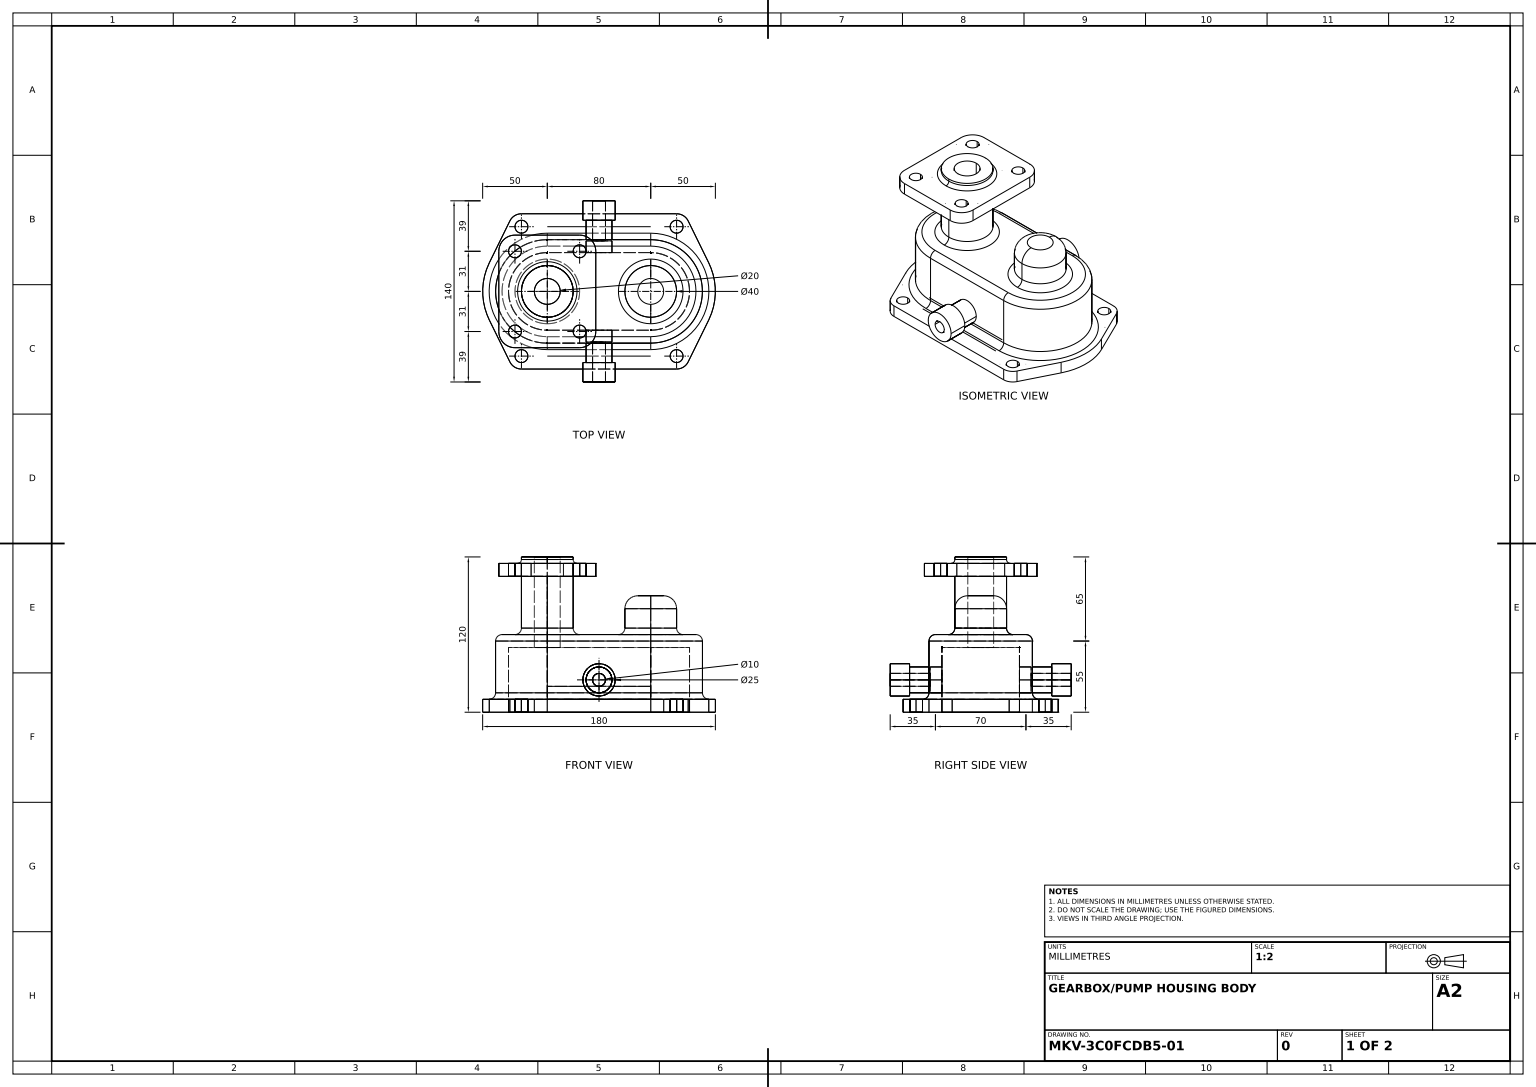
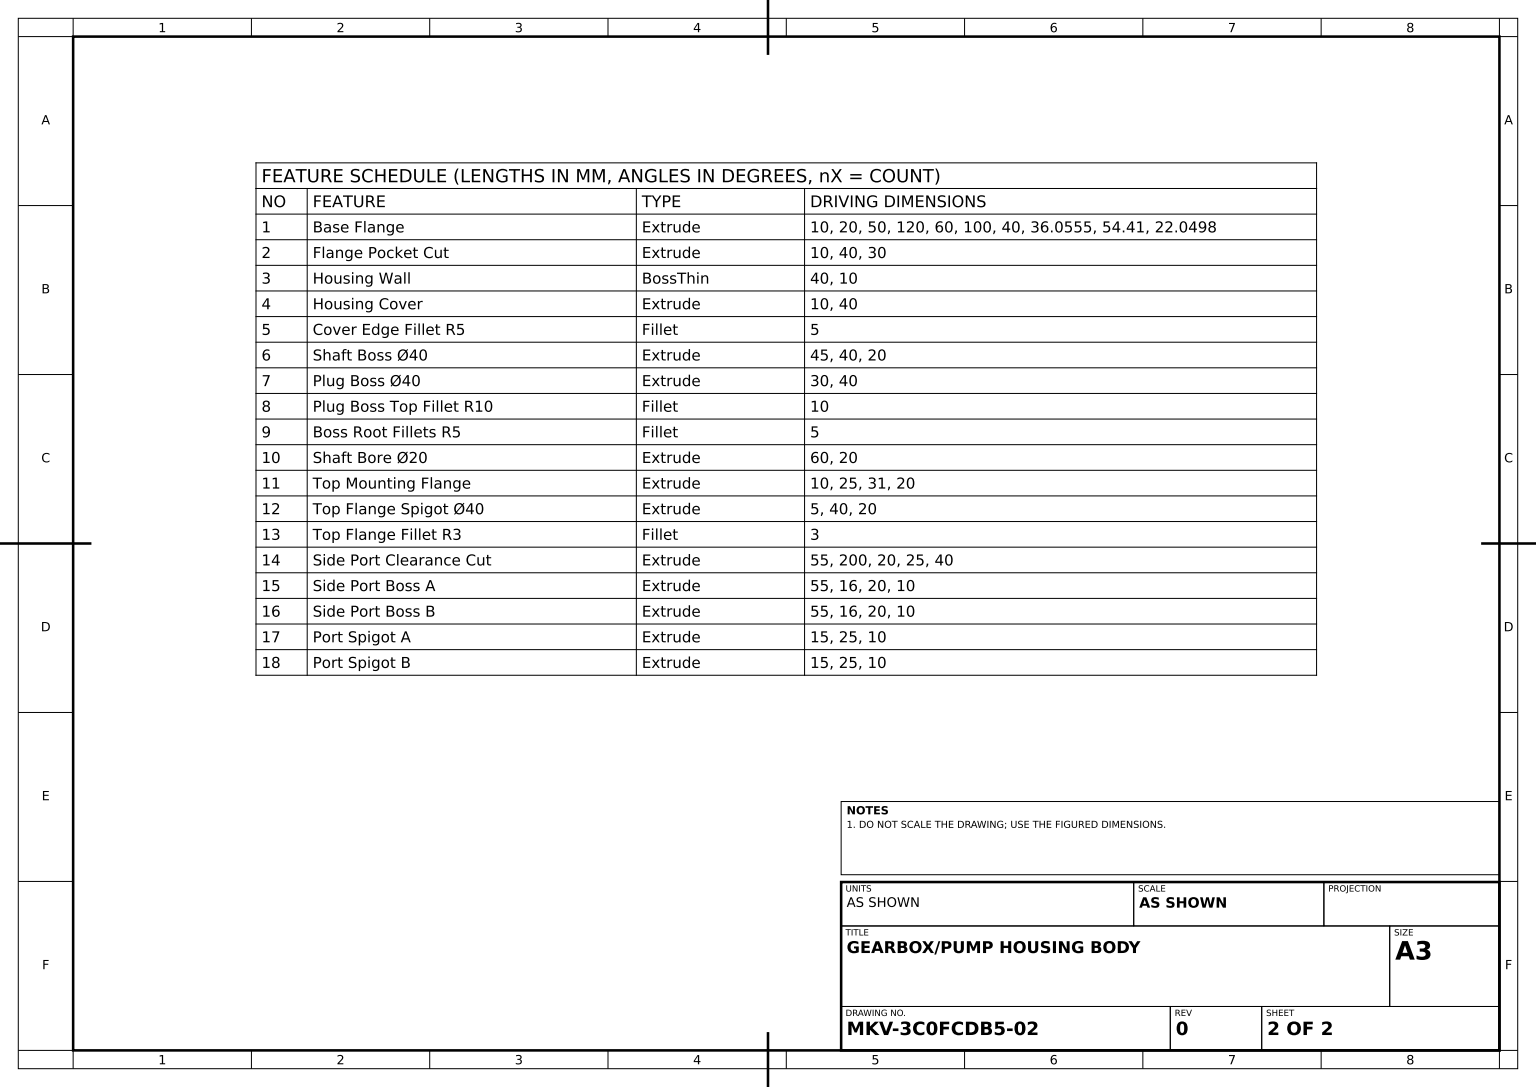
solid
v1 (-5,25,70)
v2 (5,25,70)
e1 v1 v2 CIRCLE(AX(P(0,25,70),D(0,0,1),D(1,0,0)),5)
v3 (5,25,39)
e2 v3 v2 LINE
v4 (-5,25,39)
e3 v4 v3 CIRCLE(AX(P(0,25,39),D(0,0,1),D(1,0,0)),5)
e4 v4 v1 LINE
face CYL(AX(P(0,25,39),D(0,0,1),D(1,0,0)),5) rev [e1 -e2 -e3 e4]
v5 (40,60,-35)
v6 (-40,60,-35)
e5 v5 v6 LINE
v7 (40,55,-40)
e6 v5 v7 CIRCLE(AX(P(40,55,-35),D(-1,0,0),D(0,0,1)),5)
v8 (-40,55,-40)
e7 v8 v7 LINE
e8 v6 v8 CIRCLE(AX(P(-40,55,-35),D(-1,0,0),D(0,0,1)),5)
face CYL(AX(P(-40,55,-35),D(1,0,0),D(0,0,-1)),5) [-e5 e6 -e7 -e8]
v9 (-60,10,55)
v10 (-60,0,55)
e9 v9 v10 LINE
v11 (-60,0,45)
e10 v11 v10 CIRCLE(AX(P(-60,0,50),D(0,1,0),D(0,0,1)),5)
v12 (-60,10,45)
e11 v12 v11 LINE
e12 v12 v9 CIRCLE(AX(P(-60,10,50),D(0,1,0),D(0,0,1)),5)
face CYL(AX(P(-60,10,50),D(0,-1,0),D(0,0,-1)),5) rev [e9 -e10 -e11 e12]
v13 (40,15,-40)
e13 v7 v13 LINE
v14 (40,55,40)
e14 v7 v14 CIRCLE(AX(P(40,55,0),D(0,-1,0),D(0,0,1)),40)
v15 (40,15,40)
e15 v14 v15 LINE
e16 v15 v13 CIRCLE(AX(P(40,15,0),D(0,1,0),D(0,0,1)),40)
face CYL(AX(P(40,50,0),D(0,-1,0),D(0,0,-1)),40) [-e13 e14 e15 e16]
v16 (-68.975088,0,-54.409965)
v17 (-84.875442,0,-22.049823)
e17 v16 v17 LINE
v18 (-84.875442,10,-22.049823)
e18 v18 v17 LINE
v19 (-68.975088,10,-54.409965)
e19 v19 v18 LINE
e20 v19 v16 LINE
face PLANE(AX(P(-84.875442,10,-22.049823),D(0.897508841,0,0.440996464),D(0.440996464,0,-0.897508841))) rev [e17 -e18 -e19 e20]
v20 (-40,115,23)
v21 (-40,115,-23)
e21 v20 v21 CIRCLE(AX(P(-40,115,0),D(0,-1,0),D(0,0,1)),23)
v22 (-40,118,20)
e22 v22 v20 CIRCLE(AX(P(-40,118,23),D(-1,0,0),D(0,0,1)),3)
v23 (-40,118,-20)
e23 v23 v22 CIRCLE(AX(P(-40,118,0),D(0,1,0),D(0,0,1)),20)
e24 v23 v21 CIRCLE(AX(P(-40,118,-23),D(1,0,0),D(0,0,-1)),3)
face TORUS(AX(P(-40,118,0),D(0,1,0),D(0,0,1)),23,3) rev [-e21 -e22 -e23 e24]
v24 (10,25,30)
v25 (-10,25,30)
e25 v24 v25 CIRCLE(AX(P(0,25,30),D(0,0,1),D(1,0,0)),10)
v26 (10,25,39)
e26 v24 v26 LINE
v27 (-10,25,39)
e27 v27 v26 CIRCLE(AX(P(0,25,39),D(0,0,-1),D(1,0,0)),10)
e28 v25 v27 LINE
face CYL(AX(P(0,25,-145),D(0,0,1),D(1,0,0)),10) rev [-e25 e26 -e27 -e28]
v28 (40,10,-45)
v29 (40,10,45)
e29 v28 v29 CIRCLE(AX(P(40,10,0),D(0,-1,0),D(0,0,1)),45)
v30 (-40,10,45)
e30 v29 v30 LINE
v31 (-40,10,-45)
e31 v30 v31 CIRCLE(AX(P(-40,10,0),D(0,-1,0),D(0,0,1)),45)
e32 v31 v28 LINE
v32 (60,10,-45)
v33 (60,10,-55)
e33 v32 v33 CIRCLE(AX(P(60,10,-50),D(0,1,0),D(0,0,1)),5)
e34 v33 v32 CIRCLE(AX(P(60,10,-50),D(0,1,0),D(0,0,1)),5)
e35 v9 v12 CIRCLE(AX(P(-60,10,50),D(0,1,0),D(0,0,1)),5)
v34 (60,10,45)
v35 (60,10,55)
e36 v34 v35 CIRCLE(AX(P(60,10,50),D(0,1,0),D(0,0,1)),5)
e37 v35 v34 CIRCLE(AX(P(60,10,50),D(0,1,0),D(0,0,1)),5)
v36 (60,10,60)
v37 (68.975088,10,54.409965)
e38 v36 v37 CIRCLE(AX(P(60,10,50),D(0,1,0),D(0,0,1)),10)
v38 (84.875442,10,22.049823)
e39 v37 v38 LINE
v39 (84.875442,10,-22.049823)
e40 v38 v39 CIRCLE(AX(P(40,10,0),D(0,1,0),D(0,0,1)),50)
v40 (68.975088,10,-54.409965)
e41 v39 v40 LINE
v41 (60,10,-60)
e42 v40 v41 CIRCLE(AX(P(60,10,-50),D(0,1,0),D(0,0,1)),10)
v42 (-60,10,-60)
e43 v41 v42 LINE
e44 v42 v19 CIRCLE(AX(P(-60,10,-50),D(0,1,0),D(0,0,1)),10)
v43 (-84.875442,10,22.049823)
e45 v18 v43 CIRCLE(AX(P(-40,10,0),D(0,1,0),D(0,0,1)),50)
v44 (-68.975088,10,54.409965)
e46 v43 v44 LINE
v45 (-60,10,60)
e47 v44 v45 CIRCLE(AX(P(-60,10,50),D(0,1,0),D(0,0,1)),10)
e48 v45 v36 LINE
v46 (-60,10,-55)
v47 (-60,10,-45)
e49 v46 v47 CIRCLE(AX(P(-60,10,-50),D(0,1,0),D(0,0,1)),5)
e50 v47 v46 CIRCLE(AX(P(-60,10,-50),D(0,1,0),D(0,0,1)),5)
face PLANE(AX(P(-60,10,-50),D(0,1,0),D(0,0,1))) [e29 e30 e31 e32] [-e33 -e34] [-e35 -e12] [-e36 -e37] [e38 e39 e40 e41 e42 e43 e44 e19 e45 e46 e47 e48] [-e49 -e50]
v48 (-15,105,-26)
v49 (-15,105,-36)
e51 v48 v49 CIRCLE(AX(P(-15,105,-31),D(0,1,0),D(0,0,1)),5)
e52 v49 v48 CIRCLE(AX(P(-15,105,-31),D(0,1,0),D(0,0,1)),5)
v50 (-40,105,20)
v51 (-40,105,-20)
e53 v50 v51 CIRCLE(AX(P(-40,105,0),D(0,1,0),D(0,0,1)),20)
e54 v51 v50 CIRCLE(AX(P(-40,105,0),D(0,1,0),D(0,0,1)),20)
v52 (-65,105,26)
v53 (-65,105,36)
e55 v52 v53 CIRCLE(AX(P(-65,105,31),D(0,1,0),D(0,0,1)),5)
e56 v53 v52 CIRCLE(AX(P(-65,105,31),D(0,1,0),D(0,0,1)),5)
v54 (-77.5,105,31)
v55 (-65,105,43.5)
e57 v54 v55 CIRCLE(AX(P(-65,105,31),D(0,1,0),D(0,0,1)),12.5)
v56 (-77.5,105,-31)
e58 v56 v54 LINE
v57 (-65,105,-43.5)
e59 v57 v56 CIRCLE(AX(P(-65,105,-31),D(0,1,0),D(0,0,1)),12.5)
v58 (-15,105,-43.5)
e60 v58 v57 LINE
v59 (-2.5,105,-31)
e61 v59 v58 CIRCLE(AX(P(-15,105,-31),D(0,1,0),D(0,0,1)),12.5)
v60 (-2.5,105,31)
e62 v60 v59 LINE
v61 (-15,105,43.5)
e63 v61 v60 CIRCLE(AX(P(-15,105,31),D(0,1,0),D(0,0,1)),12.5)
e64 v55 v61 LINE
v62 (-65,105,-26)
v63 (-65,105,-36)
e65 v62 v63 CIRCLE(AX(P(-65,105,-31),D(0,1,0),D(0,0,1)),5)
e66 v63 v62 CIRCLE(AX(P(-65,105,-31),D(0,1,0),D(0,0,1)),5)
v64 (-15,105,36)
v65 (-15,105,26)
e67 v64 v65 CIRCLE(AX(P(-15,105,31),D(0,1,0),D(0,0,1)),5)
e68 v65 v64 CIRCLE(AX(P(-15,105,31),D(0,1,0),D(0,0,1)),5)
face PLANE(AX(P(-65,105,-31),D(0,1,0),D(0,0,1))) rev [e51 e52] [e53 e54] [e55 e56] [-e57 -e58 -e59 -e60 -e61 -e62 -e63 -e64] [e65 e66] [e67 e68]
v66 (60,0,60)
v67 (68.975088,0,54.409965)
e69 v66 v67 CIRCLE(AX(P(60,0,50),D(0,1,0),D(0,0,1)),10)
e70 v37 v67 LINE
e71 v36 v66 LINE
face CYL(AX(P(60,10,50),D(0,-1,0),D(0,0,-1)),10) [e69 -e70 -e38 e71]
v68 (-60,0,60)
e72 v45 v68 LINE
e73 v68 v66 LINE
face PLANE(AX(P(-60,10,60),D(0,0,-1),D(-1,0,0))) rev [-e48 e72 e73 -e71]
v69 (68.975088,0,-54.409965)
e74 v40 v69 LINE
v70 (84.875442,0,-22.049823)
e75 v39 v70 LINE
e76 v70 v69 LINE
face PLANE(AX(P(84.875442,10,-22.049823),D(-0.897508841,0,0.440996464),D(0.440996464,0,0.897508841))) rev [-e74 -e41 e75 e76]
v71 (-60,0,-45)
v72 (-60,0,-55)
e77 v71 v72 CIRCLE(AX(P(-60,0,-50),D(0,1,0),D(0,0,1)),5)
e78 v47 v71 LINE
e79 v46 v72 LINE
face CYL(AX(P(-60,10,-50),D(0,-1,0),D(0,0,-1)),5) rev [-e77 -e78 e50 e79]
v73 (-40,50,10)
v74 (-40,50,-10)
e80 v73 v74 CIRCLE(AX(P(-40,50,0),D(0,1,0),D(0,0,1)),10)
v75 (-40,120,10)
e81 v75 v73 LINE
v76 (-40,120,-10)
e82 v75 v76 CIRCLE(AX(P(-40,120,0),D(0,1,0),D(0,0,1)),10)
e83 v76 v74 LINE
face CYL(AX(P(-40,105,0),D(0,-1,0),D(0,0,-1)),10) rev [-e80 -e81 e82 e83]
e84 v25 v24 CIRCLE(AX(P(0,25,30),D(0,0,1),D(1,0,0)),10)
e85 v26 v27 CIRCLE(AX(P(0,25,39),D(0,0,-1),D(1,0,0)),10)
face CYL(AX(P(0,25,-145),D(0,0,1),D(1,0,0)),10) rev [-e26 -e84 e28 -e85]
v77 (60,0,-60)
e86 v41 v77 LINE
e87 v69 v77 CIRCLE(AX(P(60,0,-50),D(0,1,0),D(0,0,1)),10)
face CYL(AX(P(60,10,-50),D(0,-1,0),D(0,0,-1)),10) [-e86 -e42 e74 e87]
v78 (-40,15,-40)
e88 v78 v31 CIRCLE(AX(P(-40,15,-45),D(1,0,0),D(0,0,-1)),5)
v79 (-40,15,40)
e89 v30 v79 CIRCLE(AX(P(-40,15,45),D(1,0,0),D(0,0,-1)),5)
e90 v78 v79 CIRCLE(AX(P(-40,15,0),D(0,1,0),D(0,0,1)),40)
face TORUS(AX(P(-40,15,0),D(0,1,0),D(0,0,1)),45,5) rev [e88 -e31 e89 -e90]
v80 (-40,120,20)
v81 (-40,120,-20)
e91 v80 v81 CIRCLE(AX(P(-40,120,0),D(0,1,0),D(0,0,1)),20)
e92 v80 v22 LINE
e93 v22 v23 CIRCLE(AX(P(-40,118,0),D(0,1,0),D(0,0,1)),20)
e94 v81 v23 LINE
face CYL(AX(P(-40,120,0),D(0,-1,0),D(0,0,-1)),20) [-e91 e92 e93 -e94]
v82 (40,60,35)
e95 v82 v5 CIRCLE(AX(P(40,60,0),D(0,1,0),D(0,0,1)),35)
e96 v14 v82 CIRCLE(AX(P(40,55,35),D(-1,0,0),D(0,0,1)),5)
face TORUS(AX(P(40,55,0),D(0,1,0),D(0,0,1)),35,5) [-e6 -e95 -e96 -e14]
v83 (40,80,-20)
v84 (40,80,20)
e97 v83 v84 CIRCLE(AX(P(40,80,0),D(0,-1,0),D(0,0,1)),20)
v85 (40,90,-10)
e98 v83 v85 CIRCLE(AX(P(40,80,-10),D(1,0,0),D(0,0,-1)),10)
v86 (40,90,10)
e99 v86 v85 CIRCLE(AX(P(40,90,0),D(0,1,0),D(0,0,1)),10)
e100 v84 v86 CIRCLE(AX(P(40,80,10),D(-1,0,0),D(0,0,1)),10)
face TORUS(AX(P(40,80,0),D(0,1,0),D(0,0,1)),10,10) [-e97 e98 -e99 -e100]
v87 (-65,115,-43.5)
v88 (-77.5,115,-31)
e101 v87 v88 CIRCLE(AX(P(-65,115,-31),D(0,1,0),D(0,0,1)),12.5)
v89 (-77.5,115,31)
e102 v88 v89 LINE
v90 (-65,115,43.5)
e103 v89 v90 CIRCLE(AX(P(-65,115,31),D(0,1,0),D(0,0,1)),12.5)
v91 (-15,115,43.5)
e104 v90 v91 LINE
v92 (-2.5,115,31)
e105 v91 v92 CIRCLE(AX(P(-15,115,31),D(0,1,0),D(0,0,1)),12.5)
v93 (-2.5,115,-31)
e106 v92 v93 LINE
v94 (-15,115,-43.5)
e107 v93 v94 CIRCLE(AX(P(-15,115,-31),D(0,1,0),D(0,0,1)),12.5)
e108 v94 v87 LINE
e109 v21 v20 CIRCLE(AX(P(-40,115,0),D(0,-1,0),D(0,0,1)),23)
v95 (-65,115,26)
v96 (-65,115,36)
e110 v95 v96 CIRCLE(AX(P(-65,115,31),D(0,1,0),D(0,0,1)),5)
e111 v96 v95 CIRCLE(AX(P(-65,115,31),D(0,1,0),D(0,0,1)),5)
v97 (-15,115,36)
v98 (-15,115,26)
e112 v97 v98 CIRCLE(AX(P(-15,115,31),D(0,1,0),D(0,0,1)),5)
e113 v98 v97 CIRCLE(AX(P(-15,115,31),D(0,1,0),D(0,0,1)),5)
v99 (-65,115,-36)
v100 (-65,115,-26)
e114 v99 v100 CIRCLE(AX(P(-65,115,-31),D(0,1,0),D(0,0,1)),5)
e115 v100 v99 CIRCLE(AX(P(-65,115,-31),D(0,1,0),D(0,0,1)),5)
v101 (-15,115,-36)
v102 (-15,115,-26)
e116 v101 v102 CIRCLE(AX(P(-15,115,-31),D(0,1,0),D(0,0,1)),5)
e117 v102 v101 CIRCLE(AX(P(-15,115,-31),D(0,1,0),D(0,0,1)),5)
face PLANE(AX(P(-65,115,-31),D(0,1,0),D(0,0,1))) [e101 e102 e103 e104 e105 e106 e107 e108] [e109 e21] [-e110 -e111] [-e112 -e113] [-e114 -e115] [-e116 -e117]
v103 (60,0,45)
e118 v34 v103 LINE
v104 (60,0,55)
e119 v104 v103 CIRCLE(AX(P(60,0,50),D(0,1,0),D(0,0,1)),5)
e120 v35 v104 LINE
face CYL(AX(P(60,10,50),D(0,-1,0),D(0,0,-1)),5) rev [e118 -e119 -e120 e37]
e121 v92 v60 LINE
e122 v93 v59 LINE
face PLANE(AX(P(-2.5,115,-31),D(-1,0,0),D(0,0,1))) rev [-e106 e121 e62 -e122]
v105 (-40,65,-20)
v106 (-40,65,20)
e123 v105 v106 CIRCLE(AX(P(-40,65,0),D(0,1,0),D(0,0,1)),20)
v107 (-40,60,-25)
e124 v105 v107 CIRCLE(AX(P(-40,65,-25),D(1,0,0),D(0,0,-1)),5)
v108 (-40,60,25)
e125 v108 v107 CIRCLE(AX(P(-40,60,0),D(0,-1,0),D(0,0,1)),25)
e126 v106 v108 CIRCLE(AX(P(-40,65,25),D(-1,0,0),D(0,0,1)),5)
face TORUS(AX(P(-40,65,0),D(0,1,0),D(0,0,1)),25,5) rev [-e123 e124 -e125 -e126]
v109 (-5,25,-39)
v110 (5,25,-39)
e127 v109 v110 CIRCLE(AX(P(0,25,-39),D(0,0,1),D(1,0,0)),5)
e128 v110 v109 CIRCLE(AX(P(0,25,-39),D(0,0,1),D(1,0,0)),5)
v111 (-10,25,-39)
v112 (10,25,-39)
e129 v111 v112 CIRCLE(AX(P(0,25,-39),D(0,0,1),D(1,0,0)),10)
e130 v112 v111 CIRCLE(AX(P(0,25,-39),D(0,0,1),D(1,0,0)),10)
face PLANE(AX(P(0,25,-39),D(0,0,1),D(1,0,0))) [-e127 -e128] [e129 e130]
v113 (-84.875442,0,22.049823)
e131 v43 v113 LINE
e132 v17 v113 CIRCLE(AX(P(-40,0,0),D(0,1,0),D(0,0,1)),50)
face CYL(AX(P(-40,10,0),D(0,-1,0),D(0,0,-1)),50) [-e131 -e45 e18 e132]
v114 (-60,0,-60)
e133 v42 v114 LINE
e134 v114 v16 CIRCLE(AX(P(-60,0,-50),D(0,1,0),D(0,0,1)),10)
face CYL(AX(P(-60,10,-50),D(0,-1,0),D(0,0,-1)),10) [e133 e134 -e20 -e44]
v115 (-40,50,30)
v116 (40,50,30)
e135 v115 v116 LINE
v117 (-40,50,-30)
e136 v117 v115 CIRCLE(AX(P(-40,50,0),D(0,1,0),D(1,0,0)),30)
v118 (40,50,-30)
e137 v118 v117 LINE
e138 v116 v118 CIRCLE(AX(P(40,50,0),D(0,1,0),D(1,0,0)),30)
e139 v74 v73 CIRCLE(AX(P(-40,50,0),D(0,1,0),D(0,0,1)),10)
face PLANE(AX(P(-40,50,0),D(0,1,0),D(0,0,1))) rev [-e135 -e136 -e137 -e138] [e139 e80]
v119 (-5,25,-70)
e140 v109 v119 LINE
v120 (5,25,-70)
e141 v119 v120 CIRCLE(AX(P(0,25,-70),D(0,0,-1),D(-1,0,0)),5)
e142 v110 v120 LINE
face CYL(AX(P(0,25,-39),D(0,0,-1),D(-1,0,0)),5) rev [e128 e140 e141 -e142]
e143 v95 v52 LINE
e144 v96 v53 LINE
face CYL(AX(P(-65,115,31),D(0,-1,0),D(0,0,-1)),5) rev [-e55 -e143 e110 e144]
e145 v76 v75 CIRCLE(AX(P(-40,120,0),D(0,1,0),D(0,0,1)),10)
face CYL(AX(P(-40,105,0),D(0,-1,0),D(0,0,-1)),10) rev [e145 e81 -e139 -e83]
v121 (40,0,30)
e146 v121 v116 LINE
v122 (-40,0,30)
e147 v122 v121 LINE
e148 v122 v115 LINE
face PLANE(AX(P(-40,0,30),D(0,0,1),D(1,0,0))) rev [e84 e25] [-e146 -e147 e148 e135]
e149 v84 v83 CIRCLE(AX(P(40,80,0),D(0,-1,0),D(0,0,1)),20)
v123 (40,65,-20)
e150 v83 v123 LINE
v124 (40,65,20)
e151 v123 v124 CIRCLE(AX(P(40,65,0),D(0,1,0),D(0,0,1)),20)
e152 v84 v124 LINE
face CYL(AX(P(40,90,0),D(0,-1,0),D(0,0,-1)),20) [e149 e150 e151 -e152]
v125 (-40,55,40)
e153 v125 v8 CIRCLE(AX(P(-40,55,0),D(0,-1,0),D(0,0,1)),40)
v126 (-40,60,35)
e154 v125 v126 CIRCLE(AX(P(-40,55,35),D(-1,0,0),D(0,0,1)),5)
e155 v6 v126 CIRCLE(AX(P(-40,60,0),D(0,1,0),D(0,0,1)),35)
face TORUS(AX(P(-40,55,0),D(0,1,0),D(0,0,1)),35,5) [-e153 e154 -e155 e8]
v127 (-10,25,-30)
e156 v111 v127 LINE
v128 (10,25,-30)
e157 v112 v128 LINE
e158 v127 v128 CIRCLE(AX(P(0,25,-30),D(0,0,-1),D(-1,0,0)),10)
face CYL(AX(P(0,25,-145),D(0,0,1),D(1,0,0)),10) rev [-e156 -e130 e157 -e158]
v129 (40,60,-25)
e159 v123 v129 CIRCLE(AX(P(40,65,-25),D(1,0,0),D(0,0,-1)),5)
e160 v124 v123 CIRCLE(AX(P(40,65,0),D(0,1,0),D(0,0,1)),20)
v130 (40,60,25)
e161 v124 v130 CIRCLE(AX(P(40,65,25),D(-1,0,0),D(0,0,1)),5)
e162 v129 v130 CIRCLE(AX(P(40,60,0),D(0,-1,0),D(0,0,1)),25)
face TORUS(AX(P(40,65,0),D(0,1,0),D(0,0,1)),25,5) rev [-e159 -e160 e161 -e162]
e163 v107 v108 CIRCLE(AX(P(-40,60,0),D(0,-1,0),D(0,0,1)),25)
e164 v106 v105 CIRCLE(AX(P(-40,65,0),D(0,1,0),D(0,0,1)),20)
face TORUS(AX(P(-40,65,0),D(0,1,0),D(0,0,1)),25,5) rev [e126 -e163 -e124 -e164]
e165 v125 v79 LINE
e166 v8 v78 LINE
face CYL(AX(P(-40,50,0),D(0,-1,0),D(0,0,-1)),40) [e90 -e165 e153 e166]
e167 v130 v129 CIRCLE(AX(P(40,60,0),D(0,-1,0),D(0,0,1)),25)
face TORUS(AX(P(40,65,0),D(0,1,0),D(0,0,1)),25,5) rev [-e167 -e161 -e151 e159]
v131 (60,0,-45)
e168 v32 v131 LINE
v132 (60,0,-55)
e169 v132 v131 CIRCLE(AX(P(60,0,-50),D(0,1,0),D(0,0,1)),5)
e170 v33 v132 LINE
face CYL(AX(P(60,10,-50),D(0,-1,0),D(0,0,-1)),5) rev [e168 -e169 -e170 e34]
v133 (-12.5,25,-55)
v134 (12.5,25,-55)
e171 v133 v134 CIRCLE(AX(P(0,25,-55),D(0,0,-1),D(-1,0,0)),12.5)
v135 (12.5,25,-70)
e172 v135 v134 LINE
v136 (-12.5,25,-70)
e173 v136 v135 CIRCLE(AX(P(0,25,-70),D(0,0,-1),D(-1,0,0)),12.5)
e174 v136 v133 LINE
face CYL(AX(P(0,25,-70),D(0,0,1),D(1,0,0)),12.5) [e171 -e172 -e173 e174]
v137 (-12.5,25,70)
v138 (-12.5,25,55)
e175 v137 v138 LINE
v139 (12.5,25,55)
e176 v138 v139 CIRCLE(AX(P(0,25,55),D(0,0,1),D(1,0,0)),12.5)
v140 (12.5,25,70)
e177 v140 v139 LINE
e178 v137 v140 CIRCLE(AX(P(0,25,70),D(0,0,1),D(1,0,0)),12.5)
face CYL(AX(P(0,25,70),D(0,0,-1),D(-1,0,0)),12.5) [e175 e176 -e177 -e178]
e179 v102 v48 LINE
e180 v101 v49 LINE
face CYL(AX(P(-15,115,-31),D(0,-1,0),D(0,0,-1)),5) rev [e116 e179 -e52 -e180]
e181 v72 v71 CIRCLE(AX(P(-60,0,-50),D(0,1,0),D(0,0,1)),5)
face CYL(AX(P(-60,10,-50),D(0,-1,0),D(0,0,-1)),5) rev [-e181 -e79 e49 e78]
e182 v140 v137 CIRCLE(AX(P(0,25,70),D(0,0,1),D(1,0,0)),12.5)
e183 v2 v1 CIRCLE(AX(P(0,25,70),D(0,0,1),D(1,0,0)),5)
face PLANE(AX(P(0,25,70),D(0,0,1),D(1,0,0))) [e178 e182] [-e1 -e183]
e184 v128 v127 CIRCLE(AX(P(0,25,-30),D(0,0,-1),D(-1,0,0)),10)
v141 (-40,0,-30)
e185 v141 v117 LINE
v142 (40,0,-30)
e186 v142 v141 LINE
e187 v142 v118 LINE
face PLANE(AX(P(-40,0,-30),D(0,0,-1),D(-1,0,0))) rev [e158 e184] [-e185 -e186 e187 e137]
e188 v10 v11 CIRCLE(AX(P(-60,0,50),D(0,1,0),D(0,0,1)),5)
face CYL(AX(P(-60,10,50),D(0,-1,0),D(0,0,-1)),5) rev [-e188 -e9 e35 e11]
face CYL(AX(P(0,25,-145),D(0,0,1),D(1,0,0)),10) rev [-e157 -e129 e156 -e184]
e189 v98 v65 LINE
e190 v97 v64 LINE
face CYL(AX(P(-15,115,31),D(0,-1,0),D(0,0,-1)),5) rev [e189 -e67 -e190 e112]
v143 (0,15,40)
e191 v79 v143 LINE
v144 (-10,25,40)
e192 v143 v144 CIRCLE(AX(P(0,25,40),D(0,0,-1),D(-1,0,0)),10)
v145 (10,25,40)
e193 v144 v145 CIRCLE(AX(P(0,25,40),D(0,0,-1),D(-1,0,0)),10)
e194 v145 v143 CIRCLE(AX(P(0,25,40),D(0,0,-1),D(-1,0,0)),10)
e195 v143 v15 LINE
e196 v14 v125 LINE
face PLANE(AX(P(-40,50,40),D(0,0,-1),D(-1,0,0))) rev [e191 e192 e193 e194 e195 -e15 e196 e165]
v146 (-68.975088,0,54.409965)
e197 v113 v146 LINE
e198 v44 v146 LINE
face PLANE(AX(P(-84.875442,10,22.049823),D(0.897508841,0,-0.440996464),D(-0.440996464,0,-0.897508841))) rev [e197 -e198 -e46 e131]
e199 v51 v105 LINE
e200 v50 v106 LINE
face CYL(AX(P(-40,105,0),D(0,-1,0),D(0,0,-1)),20) [e164 -e199 -e53 e200]
e201 v126 v82 LINE
face PLANE(AX(P(-40,60,0),D(0,1,0),D(0,0,1))) [e125 e163] [e162 e167] [e95 e5 e155 e201]
e202 v146 v68 CIRCLE(AX(P(-60,0,50),D(0,1,0),D(0,0,1)),10)
face CYL(AX(P(-60,10,50),D(0,-1,0),D(0,0,-1)),10) [-e72 -e47 e198 e202]
e203 v88 v56 LINE
e204 v89 v54 LINE
face PLANE(AX(P(-77.5,115,-31),D(1,0,0),D(0,0,-1))) rev [-e102 e203 e58 -e204]
e205 v29 v15 CIRCLE(AX(P(40,15,45),D(1,0,0),D(0,0,-1)),5)
e206 v13 v28 CIRCLE(AX(P(40,15,-45),D(1,0,0),D(0,0,-1)),5)
face TORUS(AX(P(40,15,0),D(0,1,0),D(0,0,1)),45,5) rev [-e16 -e205 -e29 -e206]
v147 (-10,25,-40)
v148 (-10,25,-55)
e207 v147 v148 LINE
v149 (10,25,-40)
e208 v147 v149 CIRCLE(AX(P(0,25,-40),D(0,0,-1),D(1,0,0)),10)
v150 (10,25,-55)
e209 v149 v150 LINE
e210 v150 v148 CIRCLE(AX(P(0,25,-55),D(0,0,1),D(1,0,0)),10)
face CYL(AX(P(0,25,-39),D(0,0,-1),D(-1,0,0)),10) [-e207 e208 e209 e210]
e211 v81 v80 CIRCLE(AX(P(-40,120,0),D(0,1,0),D(0,0,1)),20)
face PLANE(AX(P(-40,120,0),D(0,1,0),D(0,0,1))) [e91 e211] [-e82 -e145]
e212 v91 v61 LINE
e213 v90 v55 LINE
face PLANE(AX(P(-65,115,43.5),D(0,0,-1),D(-1,0,0))) rev [e64 -e212 -e104 e213]
e214 v99 v63 LINE
e215 v100 v62 LINE
face CYL(AX(P(-65,115,-31),D(0,-1,0),D(0,0,-1)),5) rev [-e214 e114 e215 -e66]
e216 v121 v142 CIRCLE(AX(P(40,0,0),D(0,1,0),D(0,0,1)),30)
face CYL(AX(P(40,0,0),D(0,1,0),D(0,0,1)),30) rev [e138 -e187 -e216 e146]
e217 v131 v132 CIRCLE(AX(P(60,0,-50),D(0,1,0),D(0,0,1)),5)
face CYL(AX(P(60,10,-50),D(0,-1,0),D(0,0,-1)),5) rev [e33 e170 -e217 -e168]
face CYL(AX(P(-40,105,0),D(0,-1,0),D(0,0,-1)),20) [e123 -e200 -e54 e199]
e218 v134 v133 CIRCLE(AX(P(0,25,-55),D(0,0,-1),D(-1,0,0)),12.5)
e219 v148 v150 CIRCLE(AX(P(0,25,-55),D(0,0,1),D(1,0,0)),10)
face PLANE(AX(P(0,25,-55),D(0,0,-1),D(-1,0,0))) rev [-e171 -e218] [-e210 -e219]
face TORUS(AX(P(-40,118,0),D(0,1,0),D(0,0,1)),23,3) rev [-e93 e22 -e109 -e24]
v151 (-10,25,55)
e220 v144 v151 LINE
v152 (10,25,55)
e221 v152 v151 CIRCLE(AX(P(0,25,55),D(0,0,1),D(1,0,0)),10)
e222 v145 v152 LINE
face CYL(AX(P(0,25,39),D(0,0,1),D(1,0,0)),10) [e220 -e221 -e222 -e193]
e223 v94 v58 LINE
e224 v87 v57 LINE
face PLANE(AX(P(-65,115,-43.5),D(0,0,1),D(1,0,0))) rev [-e108 e223 e60 -e224]
face CYL(AX(P(-65,115,-31),D(0,-1,0),D(0,0,-1)),5) rev [-e65 -e215 e115 e214]
e225 v103 v104 CIRCLE(AX(P(60,0,50),D(0,1,0),D(0,0,1)),5)
face CYL(AX(P(60,10,50),D(0,-1,0),D(0,0,-1)),5) rev [e36 e120 -e225 -e118]
e226 v3 v4 CIRCLE(AX(P(0,25,39),D(0,0,1),D(1,0,0)),5)
face PLANE(AX(P(0,25,39),D(0,0,1),D(1,0,0))) rev [e85 e27] [e226 e3]
e227 v120 v119 CIRCLE(AX(P(0,25,-70),D(0,0,-1),D(-1,0,0)),5)
face CYL(AX(P(0,25,-39),D(0,0,-1),D(-1,0,0)),5) rev [e227 -e140 e127 e142]
face CYL(AX(P(-65,115,31),D(0,-1,0),D(0,0,-1)),5) rev [e111 e143 -e56 -e144]
e228 v139 v138 CIRCLE(AX(P(0,25,55),D(0,0,1),D(1,0,0)),12.5)
face CYL(AX(P(0,25,70),D(0,0,-1),D(-1,0,0)),12.5) [-e182 e177 e228 -e175]
e229 v85 v86 CIRCLE(AX(P(40,90,0),D(0,1,0),D(0,0,1)),10)
face PLANE(AX(P(40,90,0),D(0,1,0),D(0,0,1))) [e99 e229]
e230 v135 v136 CIRCLE(AX(P(0,25,-70),D(0,0,-1),D(-1,0,0)),12.5)
face CYL(AX(P(0,25,-70),D(0,0,1),D(1,0,0)),12.5) [-e174 -e230 e172 e218]
face CYL(AX(P(-40,15,45),D(1,0,0),D(0,0,-1)),5) rev [-e89 -e30 e205 -e195 -e191]
e231 v77 v114 LINE
v153 (84.875442,0,22.049823)
e232 v153 v70 CIRCLE(AX(P(40,0,0),D(0,1,0),D(0,0,1)),50)
e233 v67 v153 LINE
e234 v141 v122 CIRCLE(AX(P(-40,0,0),D(0,1,0),D(0,0,1)),30)
face PLANE(AX(P(-60,0,-50),D(0,1,0),D(0,0,1))) rev [-e69 -e73 -e202 -e197 -e132 -e17 -e134 -e231 -e87 -e76 -e232 -e233] [e188 e10] [e119 e225] [e169 e217] [e234 e147 e216 e186] [e181 e77]
face TORUS(AX(P(40,80,0),D(0,1,0),D(0,0,1)),10,10) [e100 -e229 -e98 -e149]
face PLANE(AX(P(-60,10,-60),D(0,0,1),D(1,0,0))) rev [e86 e231 -e133 -e43]
face CYL(AX(P(-15,115,31),D(0,-1,0),D(0,0,-1)),12.5) [-e121 -e105 e212 e63]
e235 v151 v152 CIRCLE(AX(P(0,25,55),D(0,0,1),D(1,0,0)),10)
face CYL(AX(P(0,25,39),D(0,0,1),D(1,0,0)),10) [-e235 -e220 -e192 -e194 e222]
v154 (0,15,-40)
e236 v154 v78 LINE
e237 v13 v154 LINE
face CYL(AX(P(-40,15,-45),D(-1,0,0),D(0,0,1)),5) rev [-e32 -e88 -e236 -e237 e206]
e238 v149 v154 CIRCLE(AX(P(0,25,-40),D(0,0,-1),D(1,0,0)),10)
e239 v154 v147 CIRCLE(AX(P(0,25,-40),D(0,0,-1),D(1,0,0)),10)
face CYL(AX(P(0,25,-39),D(0,0,-1),D(-1,0,0)),10) [-e209 e238 e239 e207 e219]
face CYL(AX(P(-40,0,0),D(0,1,0),D(0,0,1)),30) rev [e136 -e148 -e234 e185]
face CYL(AX(P(-40,120,0),D(0,-1,0),D(0,0,-1)),20) [e23 -e92 -e211 e94]
face CYL(AX(P(-15,115,31),D(0,-1,0),D(0,0,-1)),5) rev [e190 -e68 -e189 e113]
face CYL(AX(P(-15,115,-31),D(0,-1,0),D(0,0,-1)),12.5) [e61 -e223 -e107 e122]
face CYL(AX(P(-15,115,-31),D(0,-1,0),D(0,0,-1)),5) rev [e180 -e51 -e179 e117]
e240 v38 v153 LINE
face PLANE(AX(P(84.875442,10,22.049823),D(-0.897508841,0,-0.440996464),D(-0.440996464,0,0.897508841))) rev [e70 e233 -e240 -e39]
face CYL(AX(P(-40,55,35),D(-1,0,0),D(0,0,1)),5) [-e196 e96 -e201 -e154]
face CYL(AX(P(-65,115,-31),D(0,-1,0),D(0,0,-1)),12.5) [-e101 e224 e59 -e203]
face CYL(AX(P(40,90,0),D(0,-1,0),D(0,0,-1)),20) [-e150 e97 e152 e160]
face PLANE(AX(P(0,25,-70),D(0,0,-1),D(-1,0,0))) [-e227 -e141] [e173 e230]
face CYL(AX(P(-65,115,31),D(0,-1,0),D(0,0,-1)),12.5) [-e103 e204 e57 -e213]
face PLANE(AX(P(0,25,55),D(0,0,1),D(1,0,0))) rev [e221 e235] [-e176 -e228]
face CYL(AX(P(40,10,0),D(0,-1,0),D(0,0,-1)),50) [e240 e232 -e75 -e40]
face PLANE(AX(P(-40,50,-40),D(0,0,1),D(1,0,0))) rev [e13 e237 -e238 -e208 -e239 e236 -e166 e7]
face CYL(AX(P(0,25,39),D(0,0,1),D(1,0,0)),5) rev [-e226 e2 e183 -e4]
